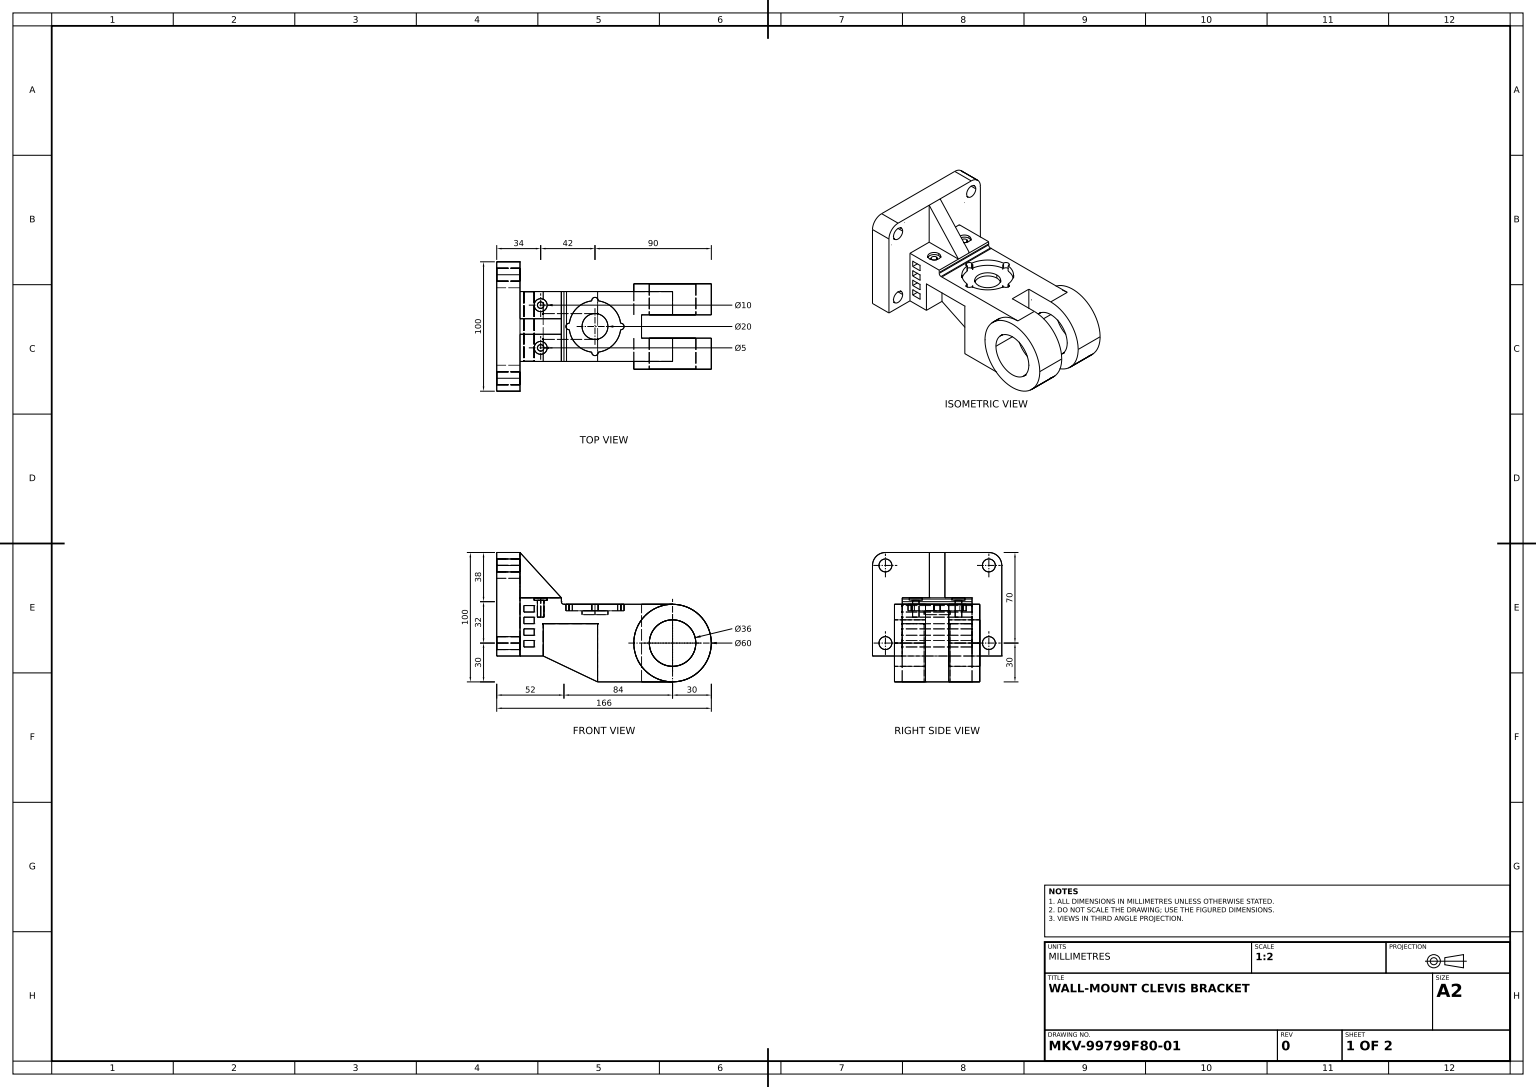
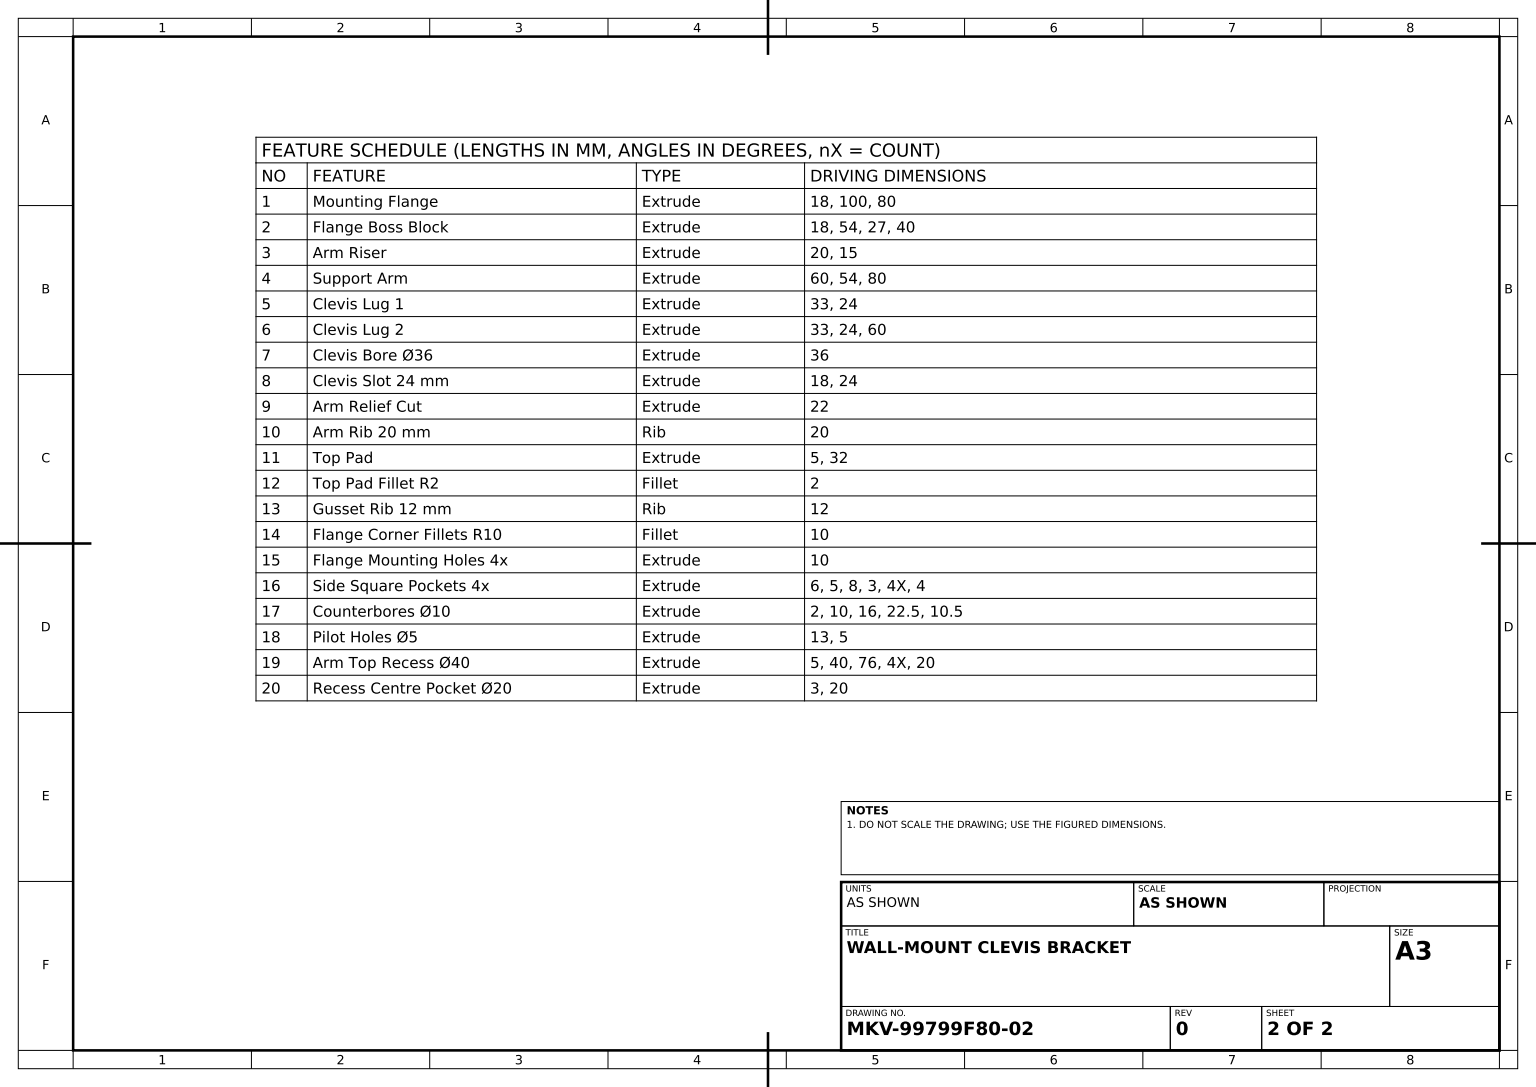
solid
v1 (36,-40,10)
v2 (36,-15,10)
e1 v1 v2 LINE
v3 (36,-15,27)
e2 v3 v2 LINE
v4 (36,-40,27)
e3 v3 v4 LINE
e4 v4 v1 LINE
face PLANE(AX(P(36,0,0),D(-1,0,0),D(0,0,1))) rev [e1 -e2 e3 e4]
v5 (21,-19,-27)
v6 (21,-24,-27)
e5 v5 v6 LINE
v7 (21,-19,27)
e6 v5 v7 LINE
v8 (21,-24,27)
e7 v8 v7 LINE
e8 v6 v8 LINE
face PLANE(AX(P(21,-19,-50),D(-1,0,0),D(0,0,1))) rev [-e5 e6 -e7 -e8]
v9 (34,5,-11.5)
v10 (34,5,-21.5)
e9 v9 v10 CIRCLE(AX(P(34,5,-16.5),D(0,1,0),D(0,0,1)),5)
v11 (34,3,-21.5)
e10 v11 v10 LINE
v12 (34,3,-11.5)
e11 v12 v11 CIRCLE(AX(P(34,3,-16.5),D(0,1,0),D(0,0,1)),5)
e12 v12 v9 LINE
face CYL(AX(P(34,3,-16.5),D(0,1,0),D(0,0,1)),5) rev [e9 -e10 -e11 e12]
v13 (29,-15,27)
v14 (21,-15,27)
e13 v13 v14 LINE
v15 (29,-15,-27)
e14 v15 v13 LINE
v16 (21,-15,-27)
e15 v16 v15 LINE
e16 v16 v14 LINE
face PLANE(AX(P(21,-15,-50),D(0,-1,0),D(0,0,-1))) rev [-e13 -e14 -e15 e16]
v17 (29,-6,-27)
v18 (29,-1,-27)
e17 v17 v18 LINE
v19 (29,-6,27)
e18 v17 v19 LINE
v20 (29,-1,27)
e19 v20 v19 LINE
e20 v18 v20 LINE
face PLANE(AX(P(29,-1,-50),D(1,0,0),D(0,0,-1))) rev [-e17 e18 -e19 -e20]
v21 (18,40,6)
v22 (50,5,6)
e21 v21 v22 LINE
v23 (18,5,6)
e22 v23 v21 LINE
e23 v23 v22 LINE
face PLANE(AX(P(83,-10,6),D(0,0,1),D(1,0,0))) [-e21 -e22 e23]
v24 (154,-30,9)
v25 (118,-30,9)
e24 v24 v25 CIRCLE(AX(P(136,-30,9),D(0,0,1),D(1,0,0)),18)
e25 v25 v24 CIRCLE(AX(P(136,-30,9),D(0,0,1),D(1,0,0)),18)
v26 (112,0,9)
v27 (136,0,9)
e26 v26 v27 LINE
v28 (166,-30,9)
e27 v28 v27 CIRCLE(AX(P(136,-30,9),D(0,0,1),D(1,0,0)),30)
v29 (136,-60,9)
e28 v29 v28 CIRCLE(AX(P(136,-30,9),D(0,0,1),D(1,0,0)),30)
v30 (112,-60,9)
e29 v30 v29 LINE
e30 v30 v26 LINE
face PLANE(AX(P(136,-30,9),D(0,0,1),D(1,0,0))) rev [e24 e25] [e26 -e27 -e28 -e29 e30]
v31 (50,2,-27)
v32 (52,0,-27)
e31 v31 v32 CIRCLE(AX(P(52,2,-27),D(0,0,1),D(0,-1,0)),2)
v33 (50,2,27)
e32 v33 v31 LINE
v34 (52,0,27)
e33 v34 v33 CIRCLE(AX(P(52,2,27),D(0,0,-1),D(-1,0,0)),2)
e34 v32 v34 LINE
face CYL(AX(P(52,2,-27),D(0,0,1),D(1,0,0)),2) rev [-e31 -e32 -e33 -e34]
v35 (95.84375,-5,-2.495112)
v36 (78.495112,-5,-19.84375)
e35 v35 v36 CIRCLE(AX(P(76,-5,0),D(0,1,0),D(0,0,1)),20)
v37 (95.84375,0,-2.495112)
e36 v35 v37 LINE
v38 (78.495112,0,-19.84375)
e37 v37 v38 CIRCLE(AX(P(76,0,0),D(0,1,0),D(0,0,1)),20)
e38 v36 v38 LINE
face CYL(AX(P(76,-5,0),D(0,1,0),D(0,0,1)),20) rev [-e35 e36 e37 -e38]
v39 (0,-30,45)
v40 (0,-30,35)
e39 v39 v40 CIRCLE(AX(P(0,-30,40),D(1,0,0),D(0,0,-1)),5)
v41 (18,-30,45)
e40 v39 v41 LINE
v42 (18,-30,35)
e41 v41 v42 CIRCLE(AX(P(18,-30,40),D(1,0,0),D(0,0,-1)),5)
e42 v40 v42 LINE
face CYL(AX(P(0,-30,40),D(1,0,0),D(0,0,-1)),5) rev [-e39 e40 e41 -e42]
e43 v10 v9 CIRCLE(AX(P(34,5,-16.5),D(0,1,0),D(0,0,1)),5)
v43 (18,5,-6)
v44 (50,5,-6)
e44 v43 v44 LINE
v45 (50,5,-27)
e45 v44 v45 LINE
v46 (18,5,-27)
e46 v45 v46 LINE
e47 v46 v43 LINE
face PLANE(AX(P(0,5,0),D(0,1,0),D(0,0,1))) [-e43 -e9] [e44 e45 e46 e47]
v47 (106,-30,33)
v48 (166,-30,33)
e48 v47 v48 CIRCLE(AX(P(136,-30,33),D(0,0,1),D(1,0,0)),30)
e49 v48 v47 CIRCLE(AX(P(136,-30,33),D(0,0,1),D(1,0,0)),30)
v49 (154,-30,33)
v50 (118,-30,33)
e50 v49 v50 CIRCLE(AX(P(136,-30,33),D(0,0,1),D(1,0,0)),18)
e51 v50 v49 CIRCLE(AX(P(136,-30,33),D(0,0,1),D(1,0,0)),18)
face PLANE(AX(P(136,-30,33),D(0,0,1),D(1,0,0))) [e48 e49] [-e50 -e51]
v51 (34,5,21.5)
v52 (34,5,11.5)
e52 v51 v52 CIRCLE(AX(P(34,5,16.5),D(0,1,0),D(0,0,1)),5)
v53 (34,3,11.5)
e53 v53 v52 LINE
v54 (34,3,21.5)
e54 v54 v53 CIRCLE(AX(P(34,3,16.5),D(0,1,0),D(0,0,1)),5)
e55 v54 v51 LINE
face CYL(AX(P(34,3,16.5),D(0,1,0),D(0,0,1)),5) rev [e52 -e53 -e54 e55]
v55 (0,30,-35)
v56 (18,30,-35)
e56 v55 v56 LINE
v57 (18,30,-45)
e57 v56 v57 CIRCLE(AX(P(18,30,-40),D(1,0,0),D(0,0,-1)),5)
v58 (0,30,-45)
e58 v58 v57 LINE
e59 v55 v58 CIRCLE(AX(P(0,30,-40),D(1,0,0),D(0,0,-1)),5)
face CYL(AX(P(0,30,-40),D(1,0,0),D(0,0,-1)),5) rev [e56 e57 -e58 -e59]
v59 (34,3,-19)
v60 (34,3,-14)
e60 v59 v60 CIRCLE(AX(P(34,3,-16.5),D(0,1,0),D(0,0,1)),2.5)
v61 (34,-10,-14)
e61 v61 v60 LINE
v62 (34,-10,-19)
e62 v62 v61 CIRCLE(AX(P(34,-10,-16.5),D(0,1,0),D(0,0,1)),2.5)
e63 v62 v59 LINE
face CYL(AX(P(34,-10,-16.5),D(0,1,0),D(0,0,1)),2.5) rev [e60 -e61 -e62 e63]
v63 (56.15625,-5,-2.495112)
v64 (56.15625,0,-2.495112)
e64 v63 v64 LINE
v65 (73.504888,-5,-19.84375)
e65 v65 v63 CIRCLE(AX(P(76,-5,0),D(0,1,0),D(0,0,1)),20)
v66 (73.504888,0,-19.84375)
e66 v65 v66 LINE
e67 v66 v64 CIRCLE(AX(P(76,0,0),D(0,1,0),D(0,0,1)),20)
face CYL(AX(P(76,-5,0),D(0,1,0),D(0,0,1)),20) rev [-e64 -e65 e66 e67]
v67 (34,-10,19)
v68 (34,3,19)
e68 v67 v68 LINE
v69 (34,3,14)
e69 v68 v69 CIRCLE(AX(P(34,3,16.5),D(0,1,0),D(0,0,1)),2.5)
v70 (34,-10,14)
e70 v70 v69 LINE
e71 v67 v70 CIRCLE(AX(P(34,-10,16.5),D(0,1,0),D(0,0,1)),2.5)
face CYL(AX(P(34,-10,16.5),D(0,1,0),D(0,0,1)),2.5) rev [e68 e69 -e70 -e71]
e72 v42 v41 CIRCLE(AX(P(18,-30,40),D(1,0,0),D(0,0,-1)),5)
e73 v40 v39 CIRCLE(AX(P(0,-30,40),D(1,0,0),D(0,0,-1)),5)
face CYL(AX(P(0,-30,40),D(1,0,0),D(0,0,-1)),5) rev [e72 -e40 -e73 e42]
v71 (0,30,45)
v72 (18,30,45)
e74 v71 v72 LINE
v73 (0,30,35)
e75 v73 v71 CIRCLE(AX(P(0,30,40),D(1,0,0),D(0,0,-1)),5)
v74 (18,30,35)
e76 v73 v74 LINE
e77 v74 v72 CIRCLE(AX(P(18,30,40),D(1,0,0),D(0,0,-1)),5)
face CYL(AX(P(0,30,40),D(1,0,0),D(0,0,-1)),5) rev [-e74 -e75 e76 e77]
e78 v36 v65 CIRCLE(AX(P(76,-5,-20),D(0,1,0),D(0,0,1)),2.5)
e79 v38 v66 CIRCLE(AX(P(76,0,-20),D(0,1,0),D(0,0,1)),2.5)
face CYL(AX(P(76,-5,-20),D(0,1,0),D(0,0,1)),2.5) rev [-e78 e38 e79 -e66]
v75 (56,-5,-2.5)
v76 (56,0,-2.5)
e80 v75 v76 LINE
v77 (56,0,2.5)
e81 v76 v77 CIRCLE(AX(P(56,0,0),D(0,1,0),D(0,0,1)),2.5)
v78 (56,-5,2.5)
e82 v78 v77 LINE
e83 v75 v78 CIRCLE(AX(P(56,-5,0),D(0,1,0),D(0,0,1)),2.5)
face CYL(AX(P(56,-5,0),D(0,1,0),D(0,0,1)),2.5) rev [e80 e81 -e82 -e83]
e84 v52 v51 CIRCLE(AX(P(34,5,16.5),D(0,1,0),D(0,0,1)),5)
e85 v53 v54 CIRCLE(AX(P(34,3,16.5),D(0,1,0),D(0,0,1)),5)
face CYL(AX(P(34,3,16.5),D(0,1,0),D(0,0,1)),5) rev [e84 -e55 -e85 e53]
e86 v70 v67 CIRCLE(AX(P(34,-10,16.5),D(0,1,0),D(0,0,1)),2.5)
face PLANE(AX(P(34,-10,16.5),D(0,1,0),D(0,0,1))) [e71 e86]
v79 (29,-33,-27)
v80 (29,-33,27)
e87 v79 v80 LINE
v81 (21,-33,-27)
e88 v81 v79 LINE
v82 (21,-33,27)
e89 v81 v82 LINE
e90 v80 v82 LINE
face PLANE(AX(P(21,-33,-50),D(0,-1,0),D(0,0,-1))) rev [-e87 -e88 e89 -e90]
v83 (136,-60,-9)
v84 (136,-60,-27)
e91 v83 v84 LINE
v85 (112,-60,-9)
e92 v83 v85 LINE
e93 v85 v30 LINE
v86 (136,-60,27)
e94 v86 v29 LINE
v87 (78,-60,27)
e95 v87 v86 LINE
v88 (78,-60,10)
e96 v87 v88 LINE
v89 (78,-60,-10)
e97 v88 v89 LINE
v90 (78,-60,-27)
e98 v89 v90 LINE
e99 v84 v90 LINE
face PLANE(AX(P(0,-60,0),D(0,1,0),D(0,0,1))) rev [-e91 e92 e93 e29 -e94 -e95 e96 e97 e98 -e99]
v91 (21,-1,27)
e100 v91 v20 LINE
v92 (21,-1,-27)
e101 v92 v91 LINE
e102 v18 v92 LINE
face PLANE(AX(P(21,-1,-50),D(0,1,0),D(0,0,1))) rev [e20 -e100 -e101 -e102]
v93 (96,-5,2.5)
v94 (96,0,2.5)
e103 v93 v94 LINE
v95 (95.84375,-5,2.495112)
e104 v95 v93 CIRCLE(AX(P(96,-5,0),D(0,1,0),D(0,0,1)),2.5)
v96 (95.84375,0,2.495112)
e105 v95 v96 LINE
e106 v96 v94 CIRCLE(AX(P(96,0,0),D(0,1,0),D(0,0,1)),2.5)
face CYL(AX(P(96,-5,0),D(0,1,0),D(0,0,1)),2.5) rev [-e103 -e104 e105 e106]
e107 v57 v56 CIRCLE(AX(P(18,30,-40),D(1,0,0),D(0,0,-1)),5)
v97 (18,30,-50)
v98 (18,40,-40)
e108 v97 v98 CIRCLE(AX(P(18,30,-40),D(1,0,0),D(0,0,1)),10)
v99 (18,40,-6)
e109 v98 v99 LINE
e110 v43 v99 LINE
v100 (18,-40,-27)
e111 v100 v46 LINE
v101 (18,-40,-50)
e112 v100 v101 LINE
e113 v101 v97 LINE
v102 (18,-30,-45)
v103 (18,-30,-35)
e114 v102 v103 CIRCLE(AX(P(18,-30,-40),D(1,0,0),D(0,0,-1)),5)
e115 v103 v102 CIRCLE(AX(P(18,-30,-40),D(1,0,0),D(0,0,-1)),5)
face PLANE(AX(P(18,0,0),D(-1,0,0),D(0,0,1))) rev [-e57 -e107] [e108 e109 -e110 -e47 -e111 e112 e113] [-e114 -e115]
v104 (0,-40,-50)
e116 v101 v104 LINE
v105 (0,30,-50)
e117 v104 v105 LINE
e118 v105 v97 LINE
face PLANE(AX(P(18,-40,-50),D(0,0,1),D(1,0,0))) rev [e116 e117 e118 -e113]
v106 (29,-28,-27)
v107 (21,-28,-27)
e119 v106 v107 LINE
v108 (29,-28,27)
e120 v106 v108 LINE
v109 (21,-28,27)
e121 v109 v108 LINE
e122 v107 v109 LINE
face PLANE(AX(P(21,-28,-50),D(0,1,0),D(0,0,1))) rev [-e119 e120 -e121 -e122]
e123 v1 v88 LINE
v110 (78,-15,10)
e124 v110 v88 LINE
e125 v2 v110 LINE
face PLANE(AX(P(83,-10,10),D(0,0,1),D(1,0,0))) [-e1 e123 -e124 -e125]
e126 v11 v12 CIRCLE(AX(P(34,3,-16.5),D(0,1,0),D(0,0,1)),5)
e127 v60 v59 CIRCLE(AX(P(34,3,-16.5),D(0,1,0),D(0,0,1)),2.5)
face PLANE(AX(P(34,3,-16.5),D(0,1,0),D(0,0,1))) [e11 e126] [-e127 -e60]
v111 (118,-30,-33)
v112 (118,-30,-9)
e128 v111 v112 LINE
v113 (154,-30,-33)
e129 v113 v111 CIRCLE(AX(P(136,-30,-33),D(0,0,1),D(1,0,0)),18)
v114 (154,-30,-9)
e130 v113 v114 LINE
e131 v114 v112 CIRCLE(AX(P(136,-30,-9),D(0,0,1),D(1,0,0)),18)
face CYL(AX(P(136,-30,-50),D(0,0,1),D(1,0,0)),18) rev [-e128 -e129 e130 e131]
e132 v108 v80 LINE
e133 v79 v106 LINE
face PLANE(AX(P(29,-28,-50),D(1,0,0),D(0,0,-1))) rev [e87 -e132 -e120 -e133]
e134 v63 v75 CIRCLE(AX(P(56,-5,0),D(0,1,0),D(0,0,1)),2.5)
e135 v64 v76 CIRCLE(AX(P(56,0,0),D(0,1,0),D(0,0,1)),2.5)
face CYL(AX(P(56,-5,0),D(0,1,0),D(0,0,1)),2.5) rev [-e134 e64 e135 -e80]
v115 (96,-5,-2.5)
v116 (96,0,-2.5)
e136 v115 v116 LINE
e137 v93 v115 CIRCLE(AX(P(96,-5,0),D(0,1,0),D(0,0,1)),2.5)
e138 v94 v116 CIRCLE(AX(P(96,0,0),D(0,1,0),D(0,0,1)),2.5)
face CYL(AX(P(96,-5,0),D(0,1,0),D(0,0,1)),2.5) rev [-e136 -e137 e103 e138]
v117 (18,30,50)
v118 (0,30,50)
e139 v117 v118 LINE
v119 (0,-40,50)
e140 v118 v119 LINE
v120 (18,-40,50)
e141 v120 v119 LINE
e142 v117 v120 LINE
face PLANE(AX(P(18,-40,50),D(0,0,-1),D(-1,0,0))) rev [e139 e140 -e141 -e142]
face CYL(AX(P(34,3,-16.5),D(0,1,0),D(0,0,1)),5) rev [e10 e43 -e12 -e126]
v121 (0,-30,-45)
v122 (0,-30,-35)
e143 v121 v122 CIRCLE(AX(P(0,-30,-40),D(1,0,0),D(0,0,-1)),5)
e144 v122 v121 CIRCLE(AX(P(0,-30,-40),D(1,0,0),D(0,0,-1)),5)
e145 v71 v73 CIRCLE(AX(P(0,30,40),D(1,0,0),D(0,0,-1)),5)
e146 v119 v104 LINE
v123 (0,40,40)
e147 v118 v123 CIRCLE(AX(P(0,30,40),D(-1,0,0),D(0,0,1)),10)
v124 (0,40,-40)
e148 v124 v123 LINE
e149 v124 v105 CIRCLE(AX(P(0,30,-40),D(-1,0,0),D(0,0,1)),10)
e150 v58 v55 CIRCLE(AX(P(0,30,-40),D(1,0,0),D(0,0,-1)),5)
face PLANE(AX(P(0,0,0),D(-1,0,0),D(0,0,1))) [e143 e144] [e145 e75] [-e146 -e140 e147 -e148 e149 -e117] [e59 e150] [e73 e39]
e151 v99 v44 LINE
face PLANE(AX(P(83,-10,-6),D(0,0,1),D(1,0,0))) rev [-e44 e110 e151]
e152 v115 v35 CIRCLE(AX(P(96,-5,0),D(0,1,0),D(0,0,1)),2.5)
e153 v116 v37 CIRCLE(AX(P(96,0,0),D(0,1,0),D(0,0,1)),2.5)
face CYL(AX(P(96,-5,0),D(0,1,0),D(0,0,1)),2.5) rev [-e152 e136 e153 -e36]
v125 (21,-6,-27)
e154 v125 v17 LINE
v126 (21,-6,27)
e155 v125 v126 LINE
e156 v19 v126 LINE
face PLANE(AX(P(21,-6,-50),D(0,-1,0),D(0,0,-1))) rev [-e18 -e154 e155 -e156]
v127 (36,-40,-10)
e157 v127 v89 LINE
v128 (36,-15,-10)
e158 v127 v128 LINE
v129 (78,-15,-10)
e159 v128 v129 LINE
e160 v129 v89 LINE
face PLANE(AX(P(83,-10,-10),D(0,0,1),D(1,0,0))) rev [-e157 e158 e159 e160]
e161 v72 v74 CIRCLE(AX(P(18,30,40),D(1,0,0),D(0,0,-1)),5)
face CYL(AX(P(0,30,40),D(1,0,0),D(0,0,-1)),5) rev [-e145 e74 e161 -e76]
v130 (78,-15,-27)
e162 v130 v129 LINE
v131 (36,-15,-27)
e163 v128 v131 LINE
e164 v130 v131 LINE
face PLANE(AX(P(56,-15,27),D(0,1,0),D(0,0,1))) rev [e162 -e159 e163 -e164]
v132 (166,-30,-9)
e165 v83 v132 CIRCLE(AX(P(136,-30,-9),D(0,0,1),D(1,0,0)),30)
v133 (106,-30,-27)
e166 v84 v133 CIRCLE(AX(P(136,-30,-27),D(0,0,-1),D(0,-1,0)),30)
v134 (106,-30,-33)
e167 v133 v134 LINE
v135 (166,-30,-33)
e168 v134 v135 CIRCLE(AX(P(136,-30,-33),D(0,0,1),D(1,0,0)),30)
e169 v132 v135 LINE
face CYL(AX(P(136,-30,-9),D(0,0,-1),D(-1,0,0)),30) [-e165 e91 e166 e167 e168 -e169]
v136 (76,-8,10)
v137 (76,-8,-10)
e170 v136 v137 CIRCLE(AX(P(76,-8,0),D(0,1,0),D(0,0,1)),10)
e171 v137 v136 CIRCLE(AX(P(76,-8,0),D(0,1,0),D(0,0,1)),10)
face PLANE(AX(P(76,-8,0),D(0,1,0),D(0,0,1))) [e170 e171]
v138 (112,0,-9)
e172 v85 v138 LINE
e173 v138 v26 LINE
face PLANE(AX(P(112,-60,-9),D(-1,0,0),D(0,0,1))) rev [e172 e173 -e30 -e93]
v139 (29,-24,-27)
e174 v6 v139 LINE
v140 (29,-24,27)
e175 v140 v8 LINE
e176 v139 v140 LINE
face PLANE(AX(P(21,-24,-50),D(0,-1,0),D(0,0,-1))) rev [-e174 e8 -e175 -e176]
e177 v122 v103 LINE
e178 v121 v102 LINE
face CYL(AX(P(0,-30,-40),D(1,0,0),D(0,0,-1)),5) rev [-e177 -e143 e178 e114]
e179 v90 v130 LINE
face PLANE(AX(P(78,-15,-50),D(1,0,0),D(0,1,0))) rev [-e162 -e179 -e98 -e160]
v141 (21,-10,27)
v142 (29,-10,27)
e180 v141 v142 LINE
v143 (21,-10,-27)
e181 v143 v141 LINE
v144 (29,-10,-27)
e182 v144 v143 LINE
e183 v144 v142 LINE
face PLANE(AX(P(21,-10,-50),D(0,1,0),D(0,0,1))) rev [-e180 -e181 -e182 e183]
v145 (76,-5,22.5)
v146 (76,0,22.5)
e184 v145 v146 LINE
v147 (78.495112,0,19.84375)
e185 v146 v147 CIRCLE(AX(P(76,0,20),D(0,1,0),D(0,0,1)),2.5)
v148 (78.495112,-5,19.84375)
e186 v148 v147 LINE
e187 v145 v148 CIRCLE(AX(P(76,-5,20),D(0,1,0),D(0,0,1)),2.5)
face CYL(AX(P(76,-5,20),D(0,1,0),D(0,0,1)),2.5) rev [e184 e185 -e186 -e187]
face CYL(AX(P(0,-30,-40),D(1,0,0),D(0,0,-1)),5) rev [e115 -e178 -e144 e177]
e188 v142 v13 LINE
e189 v15 v144 LINE
face PLANE(AX(P(29,-10,-50),D(1,0,0),D(0,0,-1))) rev [e14 -e188 -e183 -e189]
e190 v112 v114 CIRCLE(AX(P(136,-30,-9),D(0,0,1),D(1,0,0)),18)
v149 (136,0,-9)
e191 v132 v149 CIRCLE(AX(P(136,-30,-9),D(0,0,1),D(1,0,0)),30)
e192 v149 v138 LINE
face PLANE(AX(P(136,-30,-9),D(0,0,1),D(1,0,0))) [-e131 -e190] [-e172 -e92 e165 e191 e192]
v150 (36,-40,-27)
e193 v150 v100 LINE
e194 v127 v150 LINE
e195 v127 v1 LINE
v151 (18,-40,27)
e196 v4 v151 LINE
e197 v120 v151 LINE
face PLANE(AX(P(18,-40,50),D(0,1,0),D(0,0,1))) rev [-e116 -e112 -e193 -e194 e195 -e4 e196 -e197 e141 e146]
e198 v143 v16 LINE
e199 v14 v141 LINE
face PLANE(AX(P(21,-10,-50),D(-1,0,0),D(0,0,1))) rev [-e16 -e198 e181 -e199]
e200 v45 v31 LINE
e201 v22 v44 LINE
v152 (50,5,27)
e202 v152 v22 LINE
e203 v152 v33 LINE
face PLANE(AX(P(50,5,-27),D(-1,0,0),D(0,0,1))) rev [-e200 -e45 -e201 -e202 e203 e32]
e204 v82 v109 LINE
e205 v107 v81 LINE
face PLANE(AX(P(21,-28,-50),D(-1,0,0),D(0,0,1))) rev [e122 -e204 -e89 -e205]
e206 v61 v62 CIRCLE(AX(P(34,-10,-16.5),D(0,1,0),D(0,0,1)),2.5)
face PLANE(AX(P(34,-10,-16.5),D(0,1,0),D(0,0,1))) [e206 e62]
e207 v111 v113 CIRCLE(AX(P(136,-30,-33),D(0,0,1),D(1,0,0)),18)
face CYL(AX(P(136,-30,-50),D(0,0,1),D(1,0,0)),18) rev [-e130 -e207 e128 e190]
e208 v147 v96 CIRCLE(AX(P(76,0,0),D(0,1,0),D(0,0,1)),20)
e209 v148 v95 CIRCLE(AX(P(76,-5,0),D(0,1,0),D(0,0,1)),20)
face CYL(AX(P(76,-5,0),D(0,1,0),D(0,0,1)),20) rev [e208 -e105 -e209 e186]
v153 (73.504888,-5,19.84375)
v154 (73.504888,0,19.84375)
e210 v153 v154 LINE
v155 (56.15625,-5,2.495112)
e211 v155 v153 CIRCLE(AX(P(76,-5,0),D(0,1,0),D(0,0,1)),20)
v156 (56.15625,0,2.495112)
e212 v155 v156 LINE
e213 v156 v154 CIRCLE(AX(P(76,0,0),D(0,1,0),D(0,0,1)),20)
face CYL(AX(P(76,-5,0),D(0,1,0),D(0,0,1)),20) rev [-e210 -e211 e212 e213]
v157 (136,0,-27)
e214 v149 v157 LINE
e215 v135 v134 CIRCLE(AX(P(136,-30,-33),D(0,0,1),D(1,0,0)),30)
e216 v133 v157 CIRCLE(AX(P(136,-30,-27),D(0,0,-1),D(0,-1,0)),30)
face CYL(AX(P(136,-30,-9),D(0,0,-1),D(-1,0,0)),30) [-e214 -e191 e169 e215 -e167 e216]
v158 (18,40,40)
e217 v158 v117 CIRCLE(AX(P(18,30,40),D(1,0,0),D(0,0,1)),10)
e218 v123 v158 LINE
face CYL(AX(P(18,30,40),D(-1,0,0),D(0,0,1)),10) [-e147 -e139 -e217 -e218]
v159 (29,-19,-27)
e219 v139 v159 LINE
v160 (29,-19,27)
e220 v160 v140 LINE
e221 v159 v160 LINE
face PLANE(AX(P(29,-19,-50),D(1,0,0),D(0,0,-1))) rev [-e219 e176 -e220 -e221]
face PLANE(AX(P(36,-40,0),D(-0.42993358,-0.902860519,0),D(0.902860519,-0.42993358,0))) [-e123 -e195 e157 -e97]
v161 (76,-5,-10)
e222 v137 v161 LINE
v162 (76,-5,10)
e223 v161 v162 CIRCLE(AX(P(76,-5,0),D(0,1,0),D(0,0,1)),10)
e224 v136 v162 LINE
face CYL(AX(P(76,-8,0),D(0,1,0),D(0,0,1)),10) rev [-e171 e222 e223 -e224]
face CYL(AX(P(34,-10,-16.5),D(0,1,0),D(0,0,1)),2.5) rev [e127 -e63 -e206 e61]
v163 (136,0,27)
e225 v163 v27 LINE
v164 (106,-30,27)
e226 v164 v163 CIRCLE(AX(P(136,-30,27),D(0,0,-1),D(-1,0,0)),30)
e227 v164 v47 LINE
e228 v28 v48 LINE
face CYL(AX(P(136,-30,9),D(0,0,1),D(1,0,0)),30) [e27 -e225 -e226 e227 -e49 -e228]
e229 v24 v49 LINE
e230 v25 v50 LINE
face CYL(AX(P(136,-30,-50),D(0,0,1),D(1,0,0)),18) rev [e229 e50 -e230 -e24]
e231 v69 v68 CIRCLE(AX(P(34,3,16.5),D(0,1,0),D(0,0,1)),2.5)
face CYL(AX(P(34,-10,16.5),D(0,1,0),D(0,0,1)),2.5) rev [e231 -e68 -e86 e70]
e232 v78 v155 CIRCLE(AX(P(56,-5,0),D(0,1,0),D(0,0,1)),2.5)
e233 v77 v156 CIRCLE(AX(P(56,0,0),D(0,1,0),D(0,0,1)),2.5)
face CYL(AX(P(56,-5,0),D(0,1,0),D(0,0,1)),2.5) rev [-e232 e82 e233 -e212]
e234 v153 v145 CIRCLE(AX(P(76,-5,20),D(0,1,0),D(0,0,1)),2.5)
e235 v154 v146 CIRCLE(AX(P(76,0,20),D(0,1,0),D(0,0,1)),2.5)
face CYL(AX(P(76,-5,20),D(0,1,0),D(0,0,1)),2.5) rev [-e184 -e234 e210 e235]
face CYL(AX(P(136,-30,-50),D(0,0,1),D(1,0,0)),18) rev [-e25 e230 e51 -e229]
face PLANE(AX(P(34,3,16.5),D(0,1,0),D(0,0,1))) [-e231 -e69] [e54 e85]
v165 (78,-15,27)
e236 v87 v165 LINE
e237 v110 v165 LINE
face PLANE(AX(P(78,-15,-50),D(1,0,0),D(0,1,0))) rev [e124 -e96 e236 -e237]
e238 v92 v125 LINE
e239 v126 v91 LINE
face PLANE(AX(P(21,-1,-50),D(-1,0,0),D(0,0,1))) rev [-e155 -e238 e101 -e239]
e240 v165 v3 LINE
face PLANE(AX(P(56,-15,27),D(0,1,0),D(0,0,1))) rev [e237 e240 e2 e125]
e241 v159 v5 LINE
e242 v150 v131 LINE
e243 v157 v32 LINE
face PLANE(AX(P(36,-40,-27),D(0,0,1),D(0,-1,0))) rev [e154 e17 e102 e238] [e241 e5 e174 e219] [-e242 e193 e111 -e46 e200 e31 -e243 -e216 -e166 e99 e179 e164] [e15 e189 e182 e198] [e205 e88 e133 e119]
face PLANE(AX(P(136,-30,-33),D(0,0,1),D(1,0,0))) rev [-e215 -e168] [e207 e129]
e244 v21 v158 LINE
e245 v99 v21 LINE
e246 v98 v124 LINE
face PLANE(AX(P(18,40,50),D(0,-1,0),D(0,0,-1))) rev [e218 -e244 -e245 -e109 e246 e148]
e247 v86 v164 CIRCLE(AX(P(136,-30,27),D(0,0,-1),D(-1,0,0)),30)
e248 v163 v34 LINE
v166 (18,5,27)
e249 v166 v152 LINE
e250 v166 v151 LINE
e251 v7 v160 LINE
face PLANE(AX(P(36,-40,27),D(0,0,-1),D(-1,0,0))) rev [e199 e180 e188 e13] [-e240 -e236 e95 e247 e226 e248 e33 -e203 -e249 e250 -e196 -e3] [e251 e220 e175 e7] [e19 e156 e239 e100] [e132 e90 e204 e121]
face PLANE(AX(P(36,0,0),D(-1,0,0),D(0,0,1))) rev [e194 e242 -e163 -e158]
face CYL(AX(P(0,30,-40),D(1,0,0),D(0,0,-1)),5) rev [e58 e107 -e56 -e150]
face CYL(AX(P(18,30,-40),D(-1,0,0),D(0,0,1)),10) [-e108 -e118 -e149 -e246]
e252 v162 v161 CIRCLE(AX(P(76,-5,0),D(0,1,0),D(0,0,1)),10)
face CYL(AX(P(76,-8,0),D(0,1,0),D(0,0,1)),10) rev [e224 e252 -e222 -e170]
e253 v23 v166 LINE
face PLANE(AX(P(18,0,0),D(-1,0,0),D(0,0,1))) rev [-e72 -e41] [e22 e244 e217 e142 e197 -e250 -e253] [-e77 -e161]
face PLANE(AX(P(18,40,0),D(-0.738028812,-0.6747692,0),D(0.6747692,-0.738028812,0))) rev [e21 e201 -e151 e245]
face PLANE(AX(P(76,-5,10),D(0,1,0),D(0,0,1))) [-e223 -e252] [e211 e234 e187 e209 e104 e137 e152 e35 e78 e65 e134 e83 e232]
face CYL(AX(P(136,-30,9),D(0,0,1),D(1,0,0)),30) [-e48 -e227 -e247 e94 e28 e228]
face PLANE(AX(P(36,0,27),D(0,-1,0),D(0,0,-1))) rev [-e185 -e235 -e213 -e233 -e81 -e135 -e67 -e79 -e37 -e153 -e138 -e106 -e208] [e243 e34 -e248 e225 -e26 -e173 -e192 e214]
face PLANE(AX(P(21,-19,-50),D(0,1,0),D(0,0,1))) rev [e221 -e251 -e6 -e241]
face PLANE(AX(P(0,5,0),D(0,1,0),D(0,0,1))) [-e52 -e84] [-e23 e253 e249 e202]
